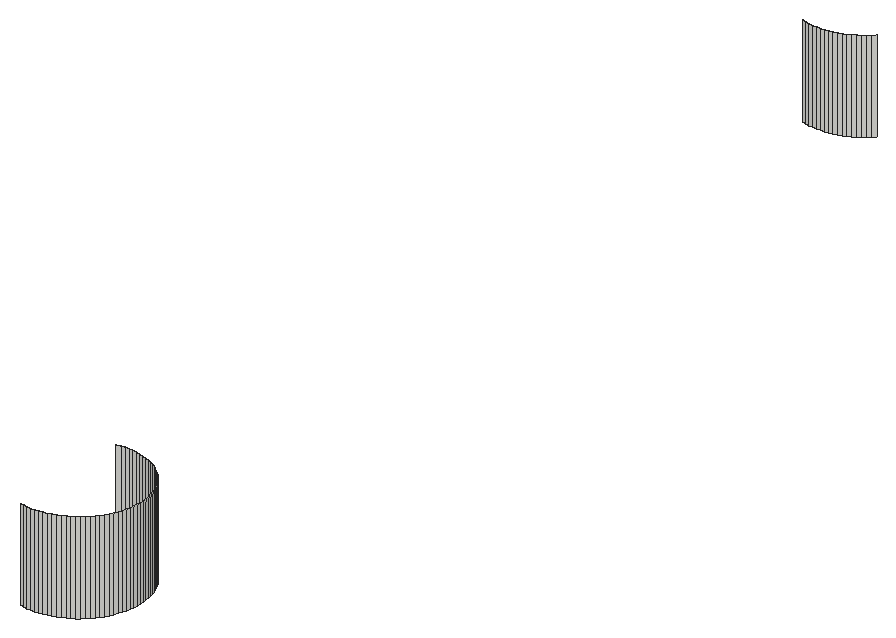
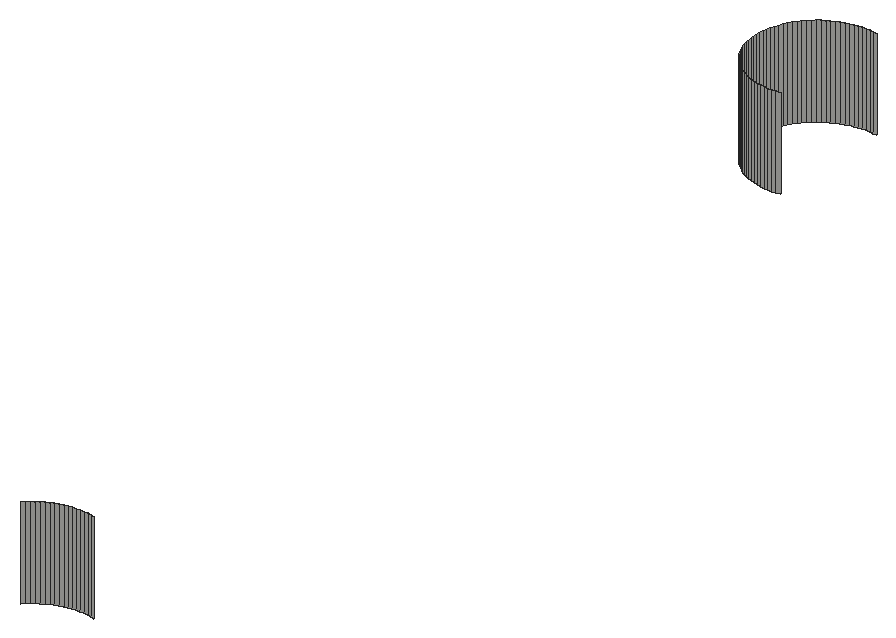
# SketchUp Ruby script. Lengths in millimetres.
U = 1.mm
M = Sketchup.active_model
def pt(a) = Geom::Point3d.new(a.map { |v| v * U })
def face(e, loops, mat)
  f = e.add_face(loops[0].map { |a| pt(a) })
  loops[1..].each { |l| e.add_face(l.map { |a| pt(a) }).erase! }
  f.material = f.back_material = mat if mat
  f
end
# faces: each face lists its corners as indices into pts; further lists are holes
def faces(e, pts, list, mat = nil) = list.each { |f| face(e, (f[0].is_a?(Array) ? f : [f]).map { |l| l.map { |i| pts[i] } }, mat) }
# xy, xz, yz: faces in a plane at the given z, y or x. An outline is a flat list of corners, or four numbers for a rectangle; further outlines are holes
def ring(l) = l.size == 4 ? [[l[0], l[1]], [l[2], l[1]], [l[2], l[3]], [l[0], l[3]]] : l.each_slice(2).to_a
def flat(e, list, mat, &to3) = list.each { |f| face(e, (f[0].is_a?(Array) ? f : [f]).map { |l| ring(l).map { |u, v| to3.(u, v) } }, mat) }
def xy(e, z, list, mat = nil) = flat(e, list, mat) { |x, y| [x, y, z] }
def xz(e, y, list, mat = nil) = flat(e, list, mat) { |x, z| [x, y, z] }
def yz(e, x, list, mat = nil) = flat(e, list, mat) { |y, z| [x, y, z] }
def lines(e, pts, list) = list.each { |a, b| e.add_line(pt(pts[a]), pt(pts[b])) }
# prism: a flat outline (further loops are holes) pulled along v
def prism(e, loops, v, mat = nil)
  f = face(e, loops, mat); d = Geom::Vector3d.new(v.map { |x| x * U })
  f.pushpull(f.normal.samedirection?(d) ? d.length : -d.length)
end
def box(e, o, s, mat = nil) = prism(e, [[o, [o[0] + s[0], o[1], o[2]], [o[0] + s[0], o[1] + s[1], o[2]], [o[0], o[1] + s[1], o[2]]]], [0, 0, s[2]], mat)
def at(x, y, z, deg = 0) = Geom::Transformation.translation(pt([x, y, z])) * Geom::Transformation.rotation(ORIGIN, Z_AXIS, deg.degrees)
def axes(o, x, y, z) = Geom::Transformation.new([*x, 0, *y, 0, *z, 0, *pt(o).to_a, 1])
def part(name) = M.definitions.add(name)
# library, detail: a bought-in or finely detailed component or shape, given as its bounding box
def library(name, o, s) = part(name).tap { |d| box(d.entities, o, s) }
def detail(e, o, s) = box(e.add_group.entities, o, s)
def put(e, d, t, mat = nil) = e.add_instance(d, t).tap { |i| i.material = mat if mat }
def group(e, t, mat = nil) = e.add_group.tap { |g| g.transformation = t; g.material = mat if mat }.entities
root = M.entities
p = [[3479,995.6,2718.2],[3479,995.6,2794],[3482.2,995.5,2794],[3482.2,995.5,2718.2],[3485.4,995.6,2794],[3485.4,995.6,2718.2],
  [3475.8,995.9,2718.2],[3475.8,995.9,2794],[3488.6,995.9,2794],[3488.6,995.9,2718.2],[3472.7,996.4,2718.2],[3472.7,996.4,2794],
  [3491.7,996.4,2794],[3491.7,996.4,2718.2],[3494.8,997.1,2794],[3494.8,997.1,2718.2],[3497.9,998,2794],[3497.9,998,2718.2],
  [3500.9,999,2794],[3500.9,999,2718.2],[3503.8,1000.3,2794],[3503.8,1000.3,2718.2],[3506.7,1001.8,2794],[3506.7,1001.8,2718.2],
  [3509.4,1003.4,2794],[3509.4,1003.4,2718.2],[3512.1,1005.2,2794],[3512.1,1005.2,2718.2],[3514.6,1007.1,2794],[3514.6,1007.1,2718.2],
  [3517,1009.2,2794],[3517,1009.2,2718.2],[3519.2,1011.5,2794],[3519.2,1011.5,2718.2],[3521.3,1013.9,2794],[3521.3,1013.9,2718.2],
  [3523.3,1016.4,2794],[3523.3,1016.4,2718.2],[3525.1,1019,2794],[3525.1,1019,2718.2],[3526.7,1021.8,2794],[3526.7,1021.8,2718.2],
  [3528.2,1024.6,2794],[3528.2,1024.6,2718.2],[3529.4,1027.6,2794],[3529.4,1027.6,2718.2],[3530.5,1030.6,2794],[3530.5,1030.6,2718.2],
  [3531.4,1033.6,2794],[3531.4,1033.6,2718.2],[3532.1,1036.7,2794],[3532.1,1036.7,2718.2],[3532.6,1039.9,2794],[3532.6,1039.9,2718.2],
  [3532.9,1043.1,2794],[3532.9,1043.1,2718.2],[3533,1046.3,2794],[3533,1046.3,2718.2],[3532.9,1049.5,2794],[3532.9,1049.5,2718.2],
  [3532.6,1052.6,2794],[3532.6,1052.6,2718.2],[3532.1,1055.8,2794],[3532.1,1055.8,2718.2],[3531.4,1058.9,2794],[3531.4,1058.9,2718.2],
  [3530.5,1062,2794],[3530.5,1062,2718.2],[3529.4,1065,2794],[3529.4,1065,2718.2],[3528.2,1067.9,2794],[3528.2,1067.9,2718.2],
  [3526.7,1070.7,2794],[3526.7,1070.7,2718.2],[3525.1,1073.5,2794],[3525.1,1073.5,2718.2],[3523.3,1076.1,2794],[3523.3,1076.1,2718.2],
  [3521.3,1078.6,2794],[3521.3,1078.6,2718.2],[3519.2,1081,2794],[3519.2,1081,2718.2],[3517,1083.3,2794],[3517,1083.3,2718.2],
  [3514.6,1085.4,2794],[3514.6,1085.4,2718.2],[3512.1,1087.4,2794],[3512.1,1087.4,2718.2],[3509.4,1089.2,2794],[3509.4,1089.2,2718.2],
  [3506.7,1090.8,2794],[3506.7,1090.8,2718.2],[3503.8,1092.2,2794],[3503.8,1092.2,2718.2],[3500.9,1093.5,2794],[3500.9,1093.5,2718.2],
  [3497.9,1094.6,2794],[3497.9,1094.6,2718.2],[3494.8,1095.5,2794],[3494.8,1095.5,2718.2],[3491.7,1096.2,2794],[3491.7,1096.2,2718.2],
  [3475.8,1096.7,2718.2],[3475.8,1096.7,2794],[3472.7,1096.2,2794],[3472.7,1096.2,2718.2],[3488.6,1096.7,2794],[3488.6,1096.7,2718.2],
  [3479,1097,2718.2],[3479,1097,2794],[3485.4,1097,2794],[3485.4,1097,2718.2],[3482.2,1097.1,2718.2],[3482.2,1097.1,2794],
  [3479,1813.2,2718.2],[3479,1813.2,2794],[3482.2,1813.1,2794],[3482.2,1813.1,2718.2],[3485.4,1813.2,2794],[3485.4,1813.2,2718.2],
  [3475.8,1813.5,2718.2],[3475.8,1813.5,2794],[3488.6,1813.5,2794],[3488.6,1813.5,2718.2],[3472.7,1814,2718.2],[3472.7,1814,2794],
  [3491.7,1814,2794],[3491.7,1814,2718.2],[3469.6,1814.7,2718.2],[3469.6,1814.7,2794],[3494.8,1814.7,2794],[3494.8,1814.7,2718.2],
  [3497.9,1815.6,2794],[3497.9,1815.6,2718.2],[3500.9,1816.7,2794],[3500.9,1816.7,2718.2],[3503.8,1818,2794],[3503.8,1818,2718.2],
  [3506.7,1819.4,2794],[3506.7,1819.4,2718.2],[3509.4,1821,2794],[3509.4,1821,2718.2],[3512.1,1822.8,2794],[3512.1,1822.8,2718.2],
  [3514.6,1824.8,2794],[3514.6,1824.8,2718.2],[3517,1826.9,2794],[3517,1826.9,2718.2],[3519.2,1829.2,2794],[3519.2,1829.2,2718.2]]
faces(root,p,[[0,1,2,3],[3,2,4,5],[6,7,1,0],[5,4,8,9],[10,11,7,6],[9,8,12,13],[13,12,14,15],[15,14,16,17],
  [17,16,18,19],[19,18,20,21],[21,20,22,23],[23,22,24,25],[25,24,26,27],[27,26,28,29],[29,28,30,31],[31,30,32,33],
  [33,32,34,35],[35,34,36,37],[37,36,38,39],[39,38,40,41],[41,40,42,43],[43,42,44,45],[45,44,46,47],[47,46,48,49],
  [49,48,50,51],[51,50,52,53],[53,52,54,55],[55,54,56,57],[57,56,58,59],[59,58,60,61],[61,60,62,63],[63,62,64,65],
  [65,64,66,67],[67,66,68,69],[69,68,70,71],[71,70,72,73],[73,72,74,75],[75,74,76,77],[77,76,78,79],[79,78,80,81],
  [81,80,82,83],[83,82,84,85],[85,84,86,87],[87,86,88,89],[89,88,90,91],[91,90,92,93],[93,92,94,95],[95,94,96,97],
  [97,96,98,99],[99,98,100,101],[102,103,104,105],[101,100,106,107],[108,109,103,102],[107,106,110,111],[112,113,109,108],[111,110,113,112],
  [114,115,116,117],[117,116,118,119],[120,121,115,114],[119,118,122,123],[124,125,121,120],[123,122,126,127],[128,129,125,124],[127,126,130,131],
  [131,130,132,133],[133,132,134,135],[135,134,136,137],[137,136,138,139],[139,138,140,141],[141,140,142,143],[143,142,144,145],[145,144,146,147],
  [147,146,148,149]])
